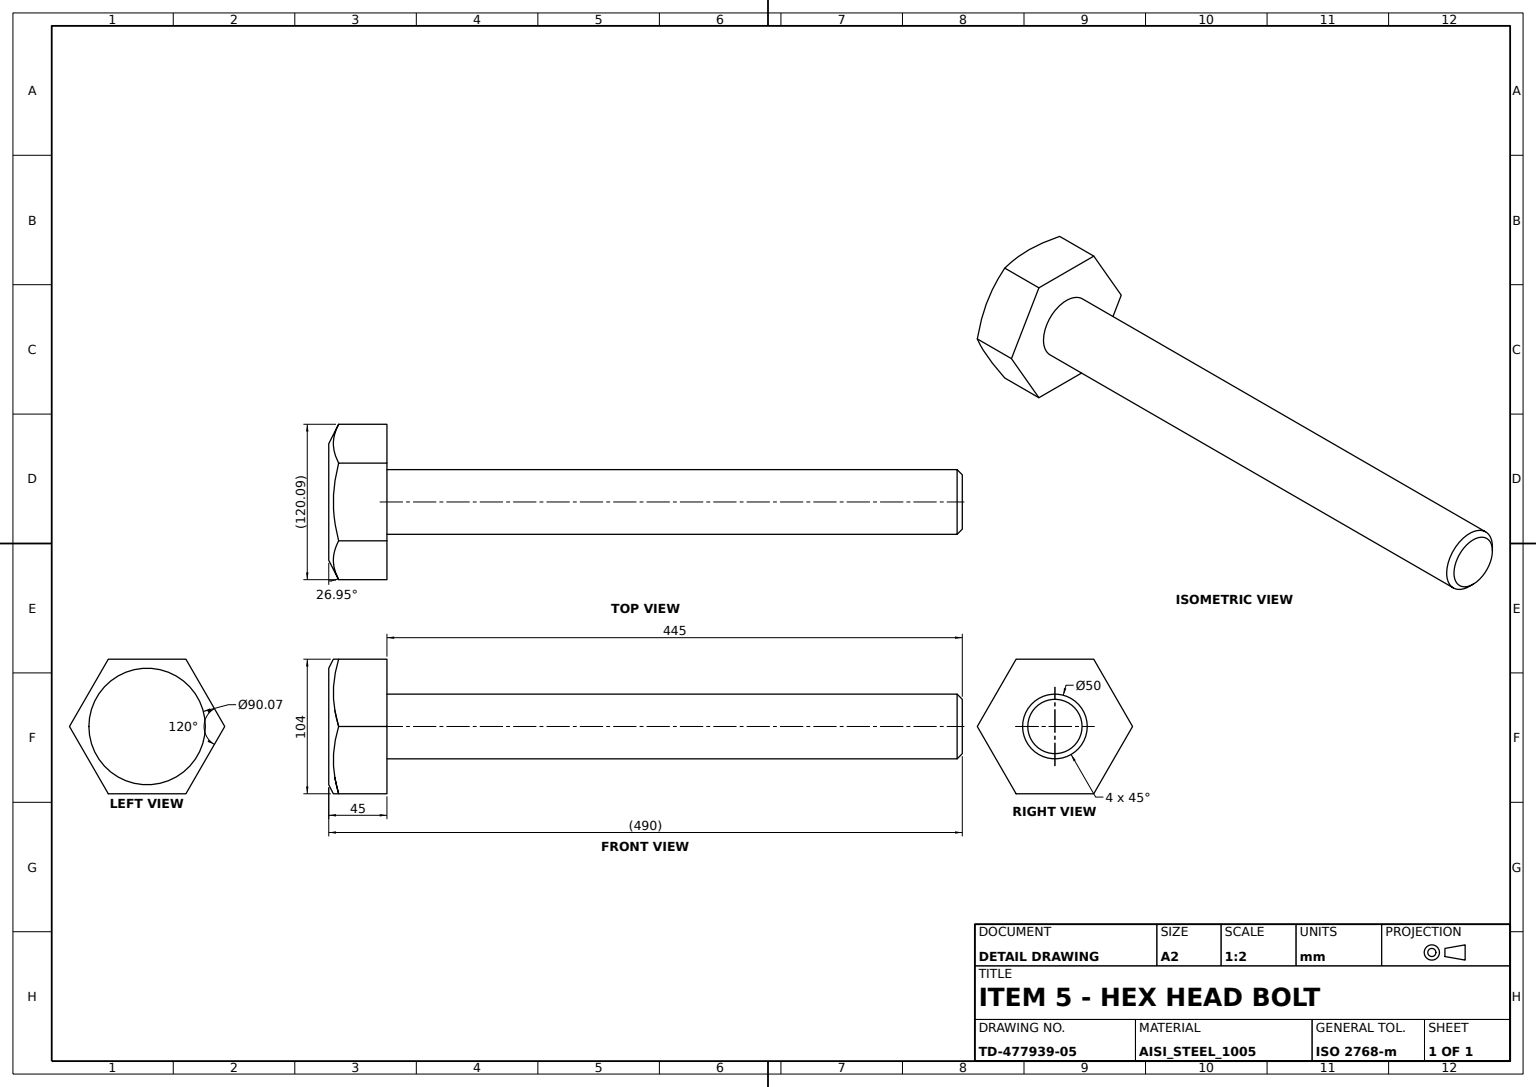
ISO-10303-21;
HEADER;
FILE_DESCRIPTION((''),'2;1');
FILE_NAME('','',(''),(''),'','','');
FILE_SCHEMA(('AUTOMOTIVE_DESIGN'));
ENDSEC;
DATA;
#1=APPLICATION_CONTEXT('');
#2=PRODUCT_CONTEXT('',#1,'mechanical');
#3=PRODUCT('','','',(#2));
#4=PRODUCT_DEFINITION_FORMATION('','',#3);
#5=PRODUCT_DEFINITION_CONTEXT('',#1,'design');
#6=PRODUCT_DEFINITION('','',#4,#5);
#7=PRODUCT_DEFINITION_SHAPE('','',#6);
#8=(LENGTH_UNIT()NAMED_UNIT(*)SI_UNIT(.MILLI.,.METRE.));
#9=(NAMED_UNIT(*)PLANE_ANGLE_UNIT()SI_UNIT($,.RADIAN.));
#10=(NAMED_UNIT(*)SI_UNIT($,.STERADIAN.)SOLID_ANGLE_UNIT());
#11=UNCERTAINTY_MEASURE_WITH_UNIT(LENGTH_MEASURE(0.005),#8,'distance_accuracy_value','');
#12=(GEOMETRIC_REPRESENTATION_CONTEXT(3)GLOBAL_UNCERTAINTY_ASSIGNED_CONTEXT((#11))GLOBAL_UNIT_ASSIGNED_CONTEXT((#8,#9,#10))REPRESENTATION_CONTEXT('',''));
#13=CARTESIAN_POINT('',(30.022214,52.,0.));
#14=VERTEX_POINT('',#13);
#15=CARTESIAN_POINT('',(60.044428,0.,0.));
#16=VERTEX_POINT('',#15);
#17=DIRECTION('',(0.5,-0.866025404,0.));
#18=VECTOR('',#17,1000.);
#19=LINE('',#13,#18);
#20=EDGE_CURVE('',#14,#16,#19,.T.);
#21=ORIENTED_EDGE('',*,*,#20,.F.);
#22=CARTESIAN_POINT('',(30.022214,52.,37.368213));
#23=VERTEX_POINT('',#22);
#24=CARTESIAN_POINT('',(30.022214,52.,45.));
#25=DIRECTION('',(0.,0.,-1.));
#26=VECTOR('',#25,1000.);
#27=LINE('',#24,#26);
#28=EDGE_CURVE('',#23,#14,#27,.T.);
#29=ORIENTED_EDGE('',*,*,#28,.F.);
#30=CARTESIAN_POINT('',(60.044428,0.,37.368213));
#31=VERTEX_POINT('',#30);
#32=CARTESIAN_POINT('',(57.580069,4.268394,38.621116));
#33=CARTESIAN_POINT('',(52.631469,12.839621,40.677346));
#34=CARTESIAN_POINT('',(46.375069,23.676025,41.642539));
#35=CARTESIAN_POINT('',(41.319536,32.432464,41.281869));
#36=CARTESIAN_POINT('',(36.232763,41.243014,40.179687));
#37=CARTESIAN_POINT('',(32.495972,47.715326,38.625895));
#38=B_SPLINE_CURVE_WITH_KNOTS('',3,(#30,#32,#33,#34,#35,#36,#37,#22),.UNSPECIFIED.,.F.,.F.,(4,1,1,1,1,4),(0.000000235,0.01505963,0.030119026,0.037648723,0.045178421,0.060237816),.UNSPECIFIED.);
#39=EDGE_CURVE('',#31,#23,#38,.T.);
#40=ORIENTED_EDGE('',*,*,#39,.F.);
#41=CARTESIAN_POINT('',(60.044428,0.,45.));
#42=LINE('',#41,#26);
#43=EDGE_CURVE('',#31,#16,#42,.T.);
#44=ORIENTED_EDGE('',*,*,#43,.T.);
#45=EDGE_LOOP('',(#21,#29,#40,#44));
#46=FACE_BOUND('',#45,.T.);
#47=DIRECTION('',(0.866025404,0.5,0.));
#48=DIRECTION('',(-0.5,0.866025404,0.));
#49=AXIS2_PLACEMENT_3D('',#24,#47,#48);
#50=PLANE('',#49);
#51=ADVANCED_FACE('',(#46),#50,.T.);
#52=ORIENTED_EDGE('',*,*,#43,.F.);
#53=CARTESIAN_POINT('',(30.022214,-52.,37.368213));
#54=VERTEX_POINT('',#53);
#55=CARTESIAN_POINT('',(32.486573,-47.731606,38.621116));
#56=CARTESIAN_POINT('',(37.435173,-39.160379,40.677346));
#57=CARTESIAN_POINT('',(43.691573,-28.323975,41.642539));
#58=CARTESIAN_POINT('',(48.747106,-19.567536,41.281869));
#59=CARTESIAN_POINT('',(53.833879,-10.756986,40.179687));
#60=CARTESIAN_POINT('',(57.57067,-4.284674,38.625895));
#61=B_SPLINE_CURVE_WITH_KNOTS('',3,(#53,#55,#56,#57,#58,#59,#60,#30),.UNSPECIFIED.,.F.,.F.,(4,1,1,1,1,4),(0.000000235,0.01505963,0.030119026,0.037648723,0.045178421,0.060237816),.UNSPECIFIED.);
#62=EDGE_CURVE('',#54,#31,#61,.T.);
#63=ORIENTED_EDGE('',*,*,#62,.F.);
#64=CARTESIAN_POINT('',(30.022214,-52.,0.));
#65=VERTEX_POINT('',#64);
#66=CARTESIAN_POINT('',(30.022214,-52.,45.));
#67=LINE('',#66,#26);
#68=EDGE_CURVE('',#54,#65,#67,.T.);
#69=ORIENTED_EDGE('',*,*,#68,.T.);
#70=DIRECTION('',(-0.5,-0.866025404,0.));
#71=VECTOR('',#70,1000.);
#72=LINE('',#15,#71);
#73=EDGE_CURVE('',#16,#65,#72,.T.);
#74=ORIENTED_EDGE('',*,*,#73,.F.);
#75=EDGE_LOOP('',(#52,#63,#69,#74));
#76=FACE_BOUND('',#75,.T.);
#77=DIRECTION('',(0.866025404,-0.5,0.));
#78=DIRECTION('',(0.5,0.866025404,0.));
#79=AXIS2_PLACEMENT_3D('',#41,#77,#78);
#80=PLANE('',#79);
#81=ADVANCED_FACE('',(#76),#80,.T.);
#82=CARTESIAN_POINT('',(-30.022214,-52.,0.));
#83=VERTEX_POINT('',#82);
#84=DIRECTION('',(-1.,0.,0.));
#85=VECTOR('',#84,1000.);
#86=LINE('',#64,#85);
#87=EDGE_CURVE('',#65,#83,#86,.T.);
#88=ORIENTED_EDGE('',*,*,#87,.F.);
#89=ORIENTED_EDGE('',*,*,#68,.F.);
#90=CARTESIAN_POINT('',(-30.022214,-52.,37.368213));
#91=VERTEX_POINT('',#90);
#92=CARTESIAN_POINT('',(-25.10567,-52.,38.618022));
#93=CARTESIAN_POINT('',(-15.083346,-52.,40.700877));
#94=CARTESIAN_POINT('',(-2.529107,-52.,41.645555));
#95=CARTESIAN_POINT('',(7.548787,-52.,41.272052));
#96=CARTESIAN_POINT('',(15.14836,-52.,40.442353));
#97=CARTESIAN_POINT('',(22.671742,-52.,39.124127));
#98=CARTESIAN_POINT('',(27.582515,-52.,37.988396));
#99=B_SPLINE_CURVE_WITH_KNOTS('',3,(#90,#92,#93,#94,#95,#96,#97,#98,#53),.UNSPECIFIED.,.F.,.F.,(4,1,1,1,1,1,4),(0.05220136,0.067372337,0.082543313,0.090128801,0.09771429,0.105299778,0.112885266),.UNSPECIFIED.);
#100=EDGE_CURVE('',#91,#54,#99,.T.);
#101=ORIENTED_EDGE('',*,*,#100,.F.);
#102=CARTESIAN_POINT('',(-30.022214,-52.,45.));
#103=LINE('',#102,#26);
#104=EDGE_CURVE('',#91,#83,#103,.T.);
#105=ORIENTED_EDGE('',*,*,#104,.T.);
#106=EDGE_LOOP('',(#88,#89,#101,#105));
#107=FACE_BOUND('',#106,.T.);
#108=DIRECTION('',(0.,-1.,0.));
#109=DIRECTION('',(1.,0.,0.));
#110=AXIS2_PLACEMENT_3D('',#66,#108,#109);
#111=PLANE('',#110);
#112=ADVANCED_FACE('',(#107),#111,.T.);
#113=CARTESIAN_POINT('',(-60.044428,0.,0.));
#114=VERTEX_POINT('',#113);
#115=VECTOR('',#48,1000.);
#116=LINE('',#82,#115);
#117=EDGE_CURVE('',#83,#114,#116,.T.);
#118=ORIENTED_EDGE('',*,*,#117,.F.);
#119=ORIENTED_EDGE('',*,*,#104,.F.);
#120=CARTESIAN_POINT('',(-60.044428,0.,37.368213));
#121=VERTEX_POINT('',#120);
#122=CARTESIAN_POINT('',(-57.580069,-4.268394,38.621116));
#123=CARTESIAN_POINT('',(-52.631469,-12.839621,40.677346));
#124=CARTESIAN_POINT('',(-46.375069,-23.676025,41.642539));
#125=CARTESIAN_POINT('',(-41.319536,-32.432464,41.281869));
#126=CARTESIAN_POINT('',(-36.232763,-41.243014,40.179687));
#127=CARTESIAN_POINT('',(-32.495972,-47.715326,38.625895));
#128=B_SPLINE_CURVE_WITH_KNOTS('',3,(#120,#122,#123,#124,#125,#126,#127,#90),.UNSPECIFIED.,.F.,.F.,(4,1,1,1,1,4),(0.000000235,0.01505963,0.030119026,0.037648723,0.045178421,0.060237816),.UNSPECIFIED.);
#129=EDGE_CURVE('',#121,#91,#128,.T.);
#130=ORIENTED_EDGE('',*,*,#129,.F.);
#131=CARTESIAN_POINT('',(-60.044428,0.,45.));
#132=LINE('',#131,#26);
#133=EDGE_CURVE('',#121,#114,#132,.T.);
#134=ORIENTED_EDGE('',*,*,#133,.T.);
#135=EDGE_LOOP('',(#118,#119,#130,#134));
#136=FACE_BOUND('',#135,.T.);
#137=DIRECTION('',(-0.866025404,-0.5,0.));
#138=AXIS2_PLACEMENT_3D('',#102,#137,#17);
#139=PLANE('',#138);
#140=ADVANCED_FACE('',(#136),#139,.T.);
#141=CARTESIAN_POINT('',(25.,0.,-441.));
#142=VERTEX_POINT('',#141);
#143=CARTESIAN_POINT('',(0.,0.,-441.));
#144=DIRECTION('',(0.,0.,1.));
#145=AXIS2_PLACEMENT_3D('',#143,#144,#109);
#146=CIRCLE('',#145,25.);
#147=EDGE_CURVE('',#142,#142,#146,.T.);
#148=ORIENTED_EDGE('',*,*,#147,.T.);
#149=EDGE_LOOP('',(#148));
#150=FACE_BOUND('',#149,.T.);
#151=CARTESIAN_POINT('',(12.5,21.650635,0.));
#152=VERTEX_POINT('',#151);
#153=CARTESIAN_POINT('',(0.,0.,0.));
#154=AXIS2_PLACEMENT_3D('',#153,#144,#78);
#155=CIRCLE('',#154,25.);
#156=EDGE_CURVE('',#152,#152,#155,.T.);
#157=ORIENTED_EDGE('',*,*,#156,.F.);
#158=EDGE_LOOP('',(#157));
#159=FACE_BOUND('',#158,.T.);
#160=CARTESIAN_POINT('',(0.,0.,-445.));
#161=AXIS2_PLACEMENT_3D('',#160,#144,#109);
#162=CYLINDRICAL_SURFACE('',#161,25.);
#163=ADVANCED_FACE('',(#150,#159),#162,.T.);
#164=ORIENTED_EDGE('',*,*,#156,.T.);
#165=EDGE_LOOP('',(#164));
#166=FACE_BOUND('',#165,.T.);
#167=CARTESIAN_POINT('',(-30.022214,52.,0.));
#168=VERTEX_POINT('',#167);
#169=VECTOR('',#109,1000.);
#170=LINE('',#167,#169);
#171=EDGE_CURVE('',#168,#14,#170,.T.);
#172=ORIENTED_EDGE('',*,*,#171,.T.);
#173=ORIENTED_EDGE('',*,*,#20,.T.);
#174=ORIENTED_EDGE('',*,*,#73,.T.);
#175=ORIENTED_EDGE('',*,*,#87,.T.);
#176=ORIENTED_EDGE('',*,*,#117,.T.);
#177=VECTOR('',#78,1000.);
#178=LINE('',#113,#177);
#179=EDGE_CURVE('',#114,#168,#178,.T.);
#180=ORIENTED_EDGE('',*,*,#179,.T.);
#181=EDGE_LOOP('',(#172,#173,#174,#175,#176,#180));
#182=FACE_BOUND('',#181,.T.);
#183=AXIS2_PLACEMENT_3D('',#153,#25,#84);
#184=PLANE('',#183);
#185=ADVANCED_FACE('',(#166,#182),#184,.T.);
#186=CARTESIAN_POINT('',(-45.033321,0.,45.));
#187=VERTEX_POINT('',#186);
#188=CARTESIAN_POINT('',(0.,0.,45.));
#189=AXIS2_PLACEMENT_3D('',#188,#25,#84);
#190=CIRCLE('',#189,45.033321);
#191=EDGE_CURVE('',#187,#187,#190,.T.);
#192=ORIENTED_EDGE('',*,*,#191,.F.);
#193=EDGE_LOOP('',(#192));
#194=FACE_BOUND('',#193,.T.);
#195=PLANE('',#189);
#196=ADVANCED_FACE('',(#194),#195,.F.);
#197=ORIENTED_EDGE('',*,*,#39,.T.);
#198=CARTESIAN_POINT('',(-30.022214,52.,37.368213));
#199=VERTEX_POINT('',#198);
#200=CARTESIAN_POINT('',(-25.10567,52.,38.618022));
#201=CARTESIAN_POINT('',(-15.083346,52.,40.700877));
#202=CARTESIAN_POINT('',(-2.529107,52.,41.645555));
#203=CARTESIAN_POINT('',(7.548787,52.,41.272052));
#204=CARTESIAN_POINT('',(15.14836,52.,40.442353));
#205=CARTESIAN_POINT('',(22.671742,52.,39.124127));
#206=CARTESIAN_POINT('',(27.582515,52.,37.988396));
#207=B_SPLINE_CURVE_WITH_KNOTS('',3,(#198,#200,#201,#202,#203,#204,#205,#206,#22),.UNSPECIFIED.,.F.,.F.,(4,1,1,1,1,1,4),(0.05220136,0.067372337,0.082543313,0.090128801,0.09771429,0.105299778,0.112885266),.UNSPECIFIED.);
#208=EDGE_CURVE('',#23,#199,#207,.F.);
#209=ORIENTED_EDGE('',*,*,#208,.T.);
#210=CARTESIAN_POINT('',(-32.486573,47.731606,38.621116));
#211=CARTESIAN_POINT('',(-37.435173,39.160379,40.677346));
#212=CARTESIAN_POINT('',(-43.691573,28.323975,41.642539));
#213=CARTESIAN_POINT('',(-48.747106,19.567536,41.281869));
#214=CARTESIAN_POINT('',(-53.833879,10.756986,40.179687));
#215=CARTESIAN_POINT('',(-57.57067,4.284674,38.625895));
#216=B_SPLINE_CURVE_WITH_KNOTS('',3,(#198,#210,#211,#212,#213,#214,#215,#120),.UNSPECIFIED.,.F.,.F.,(4,1,1,1,1,4),(0.000000235,0.01505963,0.030119026,0.037648723,0.045178421,0.060237816),.UNSPECIFIED.);
#217=EDGE_CURVE('',#199,#121,#216,.T.);
#218=ORIENTED_EDGE('',*,*,#217,.T.);
#219=ORIENTED_EDGE('',*,*,#129,.T.);
#220=ORIENTED_EDGE('',*,*,#100,.T.);
#221=ORIENTED_EDGE('',*,*,#62,.T.);
#222=EDGE_LOOP('',(#197,#209,#218,#219,#220,#221));
#223=FACE_BOUND('',#222,.T.);
#224=ORIENTED_EDGE('',*,*,#191,.T.);
#225=EDGE_LOOP('',(#224));
#226=FACE_BOUND('',#225,.T.);
#227=CONICAL_SURFACE('',#189,45.033320997,1.100443924);
#228=ADVANCED_FACE('',(#223,#226),#227,.T.);
#229=CARTESIAN_POINT('',(21.,0.,-445.));
#230=VERTEX_POINT('',#229);
#231=CIRCLE('',#161,21.);
#232=EDGE_CURVE('',#230,#230,#231,.F.);
#233=ORIENTED_EDGE('',*,*,#232,.T.);
#234=EDGE_LOOP('',(#233));
#235=FACE_BOUND('',#234,.T.);
#236=PLANE('',#161);
#237=ADVANCED_FACE('',(#235),#236,.F.);
#238=ORIENTED_EDGE('',*,*,#147,.F.);
#239=EDGE_LOOP('',(#238));
#240=FACE_BOUND('',#239,.T.);
#241=ORIENTED_EDGE('',*,*,#232,.F.);
#242=EDGE_LOOP('',(#241));
#243=FACE_BOUND('',#242,.T.);
#244=CONICAL_SURFACE('',#145,25.,0.785398163);
#245=ADVANCED_FACE('',(#240,#243),#244,.T.);
#246=ORIENTED_EDGE('',*,*,#171,.F.);
#247=CARTESIAN_POINT('',(-30.022214,52.,45.));
#248=LINE('',#247,#26);
#249=EDGE_CURVE('',#199,#168,#248,.T.);
#250=ORIENTED_EDGE('',*,*,#249,.F.);
#251=ORIENTED_EDGE('',*,*,#208,.F.);
#252=ORIENTED_EDGE('',*,*,#28,.T.);
#253=EDGE_LOOP('',(#246,#250,#251,#252));
#254=FACE_BOUND('',#253,.T.);
#255=DIRECTION('',(0.,1.,0.));
#256=AXIS2_PLACEMENT_3D('',#247,#255,#84);
#257=PLANE('',#256);
#258=ADVANCED_FACE('',(#254),#257,.T.);
#259=ORIENTED_EDGE('',*,*,#217,.F.);
#260=ORIENTED_EDGE('',*,*,#249,.T.);
#261=ORIENTED_EDGE('',*,*,#179,.F.);
#262=ORIENTED_EDGE('',*,*,#133,.F.);
#263=EDGE_LOOP('',(#259,#260,#261,#262));
#264=FACE_BOUND('',#263,.T.);
#265=DIRECTION('',(-0.866025404,0.5,0.));
#266=AXIS2_PLACEMENT_3D('',#131,#265,#70);
#267=PLANE('',#266);
#268=ADVANCED_FACE('',(#264),#267,.T.);
#269=CLOSED_SHELL('',(#51,#81,#112,#140,#163,#185,#196,#228,#237,#245,#258,#268));
#270=MANIFOLD_SOLID_BREP('',#269);
#271=ADVANCED_BREP_SHAPE_REPRESENTATION('',(#270),#12);
#272=SHAPE_DEFINITION_REPRESENTATION(#7,#271);
ENDSEC;
END-ISO-10303-21;
